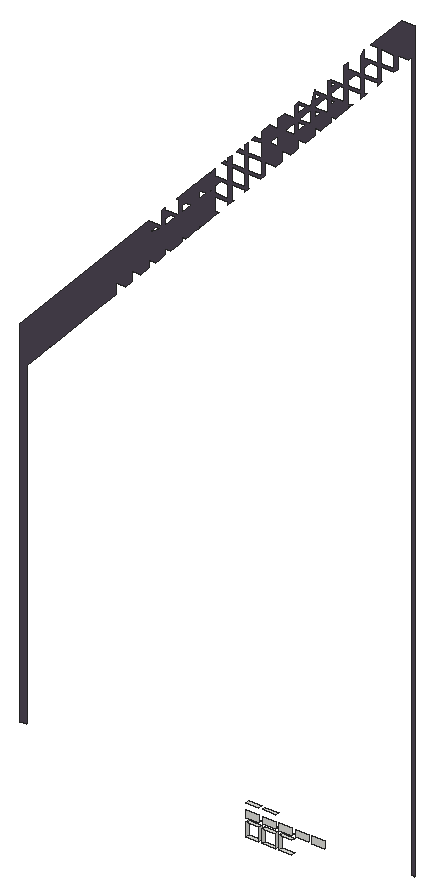
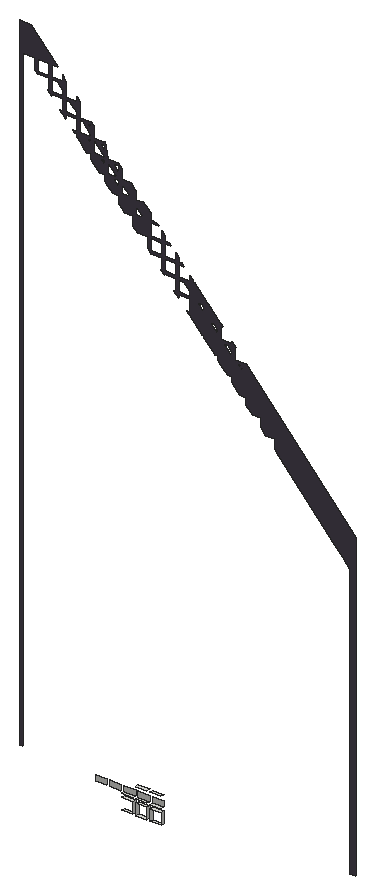
# SketchUp Ruby script. Lengths in inches.
U = 1.inch
M = Sketchup.active_model
def pt(a) = Geom::Point3d.new(a.map { |v| v * U })
def face(e, loops, mat)
  f = e.add_face(loops[0].map { |a| pt(a) })
  loops[1..].each { |l| e.add_face(l.map { |a| pt(a) }).erase! }
  f.material = f.back_material = mat if mat
  f
end
# faces: each face lists its corners as indices into pts; further lists are holes
def faces(e, pts, list, mat = nil) = list.each { |f| face(e, (f[0].is_a?(Array) ? f : [f]).map { |l| l.map { |i| pts[i] } }, mat) }
# xy, xz, yz: faces in a plane at the given z, y or x. An outline is a flat list of corners, or four numbers for a rectangle; further outlines are holes
def ring(l) = l.size == 4 ? [[l[0], l[1]], [l[2], l[1]], [l[2], l[3]], [l[0], l[3]]] : l.each_slice(2).to_a
def flat(e, list, mat, &to3) = list.each { |f| face(e, (f[0].is_a?(Array) ? f : [f]).map { |l| ring(l).map { |u, v| to3.(u, v) } }, mat) }
def xy(e, z, list, mat = nil) = flat(e, list, mat) { |x, y| [x, y, z] }
def xz(e, y, list, mat = nil) = flat(e, list, mat) { |x, z| [x, y, z] }
def yz(e, x, list, mat = nil) = flat(e, list, mat) { |y, z| [x, y, z] }
def lines(e, pts, list) = list.each { |a, b| e.add_line(pt(pts[a]), pt(pts[b])) }
# prism: a flat outline (further loops are holes) pulled along v
def prism(e, loops, v, mat = nil)
  f = face(e, loops, mat); d = Geom::Vector3d.new(v.map { |x| x * U })
  f.pushpull(f.normal.samedirection?(d) ? d.length : -d.length)
end
def box(e, o, s, mat = nil) = prism(e, [[o, [o[0] + s[0], o[1], o[2]], [o[0] + s[0], o[1] + s[1], o[2]], [o[0], o[1] + s[1], o[2]]]], [0, 0, s[2]], mat)
def at(x, y, z, deg = 0) = Geom::Transformation.translation(pt([x, y, z])) * Geom::Transformation.rotation(ORIGIN, Z_AXIS, deg.degrees)
def axes(o, x, y, z) = Geom::Transformation.new([*x, 0, *y, 0, *z, 0, *pt(o).to_a, 1])
def part(name) = M.definitions.add(name)
# library, detail: a bought-in or finely detailed component or shape, given as its bounding box
def library(name, o, s) = part(name).tap { |d| box(d.entities, o, s) }
def detail(e, o, s) = box(e.add_group.entities, o, s)
def put(e, d, t, mat = nil) = e.add_instance(d, t).tap { |i| i.material = mat if mat }
def group(e, t, mat = nil) = e.add_group.tap { |g| g.transformation = t; g.material = mat if mat }.entities
root = M.entities
M.materials.add("[Color M06]").color = [79, 71, 84]
xy(root,259.684,[[1357.054,480.141,1359.367,480.766],[1359.966,480.141,1362.279,480.766],[1362.879,480.141,1365.191,480.766]])
xy(root,261.996,[[1357.054,480.141,1359.367,480.766],[1359.966,480.141,1362.279,480.766],[1362.879,480.141,1365.191,480.766]])
xy(root,262.728,[[1357.083,480.141,1359.396,480.766],[1359.995,480.141,1362.308,480.766],[1362.908,480.141,1365.22,480.766]])
xy(root,265.041,[[1357.083,480.141,1359.396,480.766],[1359.995,480.141,1362.308,480.766]])
xz(root,480.141,[[1357.083,262.728,1359.396,263.889],[1359.995,262.728,1362.308,263.889],[1362.908,262.728,1365.22,263.889],[1365.82,262.728,1368.132,263.889],[1368.732,262.728,1371.044,263.889]])
xz(root,480.141,[[[1317.439,263.889,1318.577,263.889,1318.577,320.238,1319.662,321.395,1320.193,321.962,1322.574,324.502,1322.574,324.774,1322.829,324.774,1331.31,333.822,1333.374,336.024,1334.222,336.929,1334.222,338.837,1336.01,338.837,1337.134,340.036,1337.134,341.649,1338.646,341.649,1340.046,343.143,1340.046,344.462,1341.282,344.462,1341.751,344.962,1342.359,345.61,1342.958,346.25,1342.958,347.274,1343.918,347.274,1344.387,347.774,1345.271,348.717,1345.87,349.357,1345.87,350.087,1346.554,350.087,1347.023,350.587,1348.183,351.824,1348.782,352.464,1348.782,352.899,1349.19,352.899,1349.659,353.399,1351.095,354.931,1351.694,355.571,1351.694,355.712,1351.826,355.712,1352.295,356.212,1351.694,356.212,1351.694,358.524,1354.007,358.524,1354.007,358.038,1354.931,359.024,1354.606,359.024,1354.606,361.337,1356.919,361.337,1356.919,361.145,1357.567,361.837,1357.518,361.837,1357.518,364.149,1359.735,364.149,1360.43,364.891,1360.43,366.962,1362.371,366.962,1363.342,367.998,1363.342,369.774,1365.007,369.774,1365.476,370.274,1365.655,370.466,1366.254,371.105,1366.254,372.587,1367.643,372.587,1368.112,373.087,1368.567,373.573,1369.167,374.212,1369.167,375.399,1370.279,375.399,1370.689,375.837,1371.479,376.679,1372.079,377.319,1372.079,378.149,1372.857,378.149,1373.267,378.587,1374.391,379.786,1374.991,380.426,1374.991,380.899,1375.434,380.899,1375.844,381.337,1374.991,381.337,1374.991,383.649,1377.303,383.649,1377.303,382.893,1377.903,383.533,1377.903,383.649,1378.012,383.649,1378.101,383.746,1378.422,384.087,1377.903,384.087,1377.903,386.399,1380.215,386.399,1380.215,386,1380.999,386.837,1380.815,386.837,1380.815,389.149,1383.127,389.149,1383.127,389.107,1383.727,389.747,1383.727,391.899,1385.744,391.899,1386.175,392.359,1386.175,263.889,1386.751,263.889,1386.751,397.749,1384.501,397.749,1378.995,391.899,1380.215,391.899,1380.215,389.587,1377.903,389.587,1377.903,390.739,1377.303,390.102,1377.303,389.587,1376.818,389.587,1376.406,389.149,1377.303,389.149,1377.303,386.837,1374.991,386.837,1374.991,387.645,1374.391,387.008,1374.391,386.837,1374.229,386.837,1373.818,386.399,1374.391,386.399,1374.391,384.087,1372.079,384.087,1372.079,384.552,1371.229,383.649,1371.479,383.649,1371.479,381.337,1369.167,381.337,1369.167,381.458,1368.567,380.821,1368.567,378.587,1366.464,378.587,1365.655,377.727,1365.655,375.837,1363.875,375.837,1363.463,375.399,1363.342,375.271,1362.743,374.634,1362.743,373.087,1361.287,373.087,1360.816,372.587,1360.43,372.177,1359.831,371.54,1359.831,370.274,1358.639,370.274,1358.169,369.774,1359.831,369.774,1359.831,367.462,1357.518,367.462,1357.518,369.083,1356.919,368.447,1356.919,367.462,1355.992,367.462,1355.521,366.962,1356.919,366.962,1356.919,364.649,1354.606,364.649,1354.606,365.99,1354.007,365.353,1354.007,364.649,1353.344,364.649,1352.874,364.149,1354.007,364.149,1354.007,361.837,1351.694,361.837,1351.694,362.896,1351.095,362.259,1351.095,361.837,1350.697,361.837,1350.226,361.337,1348.782,359.803,1348.183,359.166,1348.183,359.024,1348.05,359.024,1347.579,358.524,1345.87,356.709,1344.932,355.712,1345.271,355.712,1345.271,353.399,1342.958,353.399,1342.958,353.615,1342.284,352.899,1342.359,352.899,1342.359,350.587,1340.107,350.587,1317.439,326.504],[1354.606,361.837,1356.919,364.149],[1357.518,364.649,1359.831,366.962],[1380.815,389.587,1383.127,391.899],[1377.903,386.837,1377.903,387.983,1379,389.149,1380.215,389.149,1380.215,386.837],[1351.694,359.024,1351.694,360.14,1352.82,361.337,1354.007,361.337,1354.007,359.024],[1374.991,384.087,1374.991,384.89,1376.412,386.399,1377.303,386.399,1377.303,384.087],[1372.079,381.337,1372.079,381.796,1373.823,383.649,1374.391,383.649,1374.391,381.337],[1369.167,378.587,1369.167,378.702,1371.234,380.899,1371.479,380.899,1371.479,378.587],[1366.469,375.837,1368.567,378.065,1368.567,375.837],[1340.046,347.774,1340.046,348.768,1341.282,350.087,1342.231,350.087,1340.054,347.774],[1363.881,373.087,1365.655,374.972,1365.655,373.087],[1342.958,350.86,1342.958,351.875,1343.918,352.899,1344.878,352.899],[1361.233,370.274,1362.743,371.878,1362.743,370.274],[1345.87,353.953,1345.87,354.982,1346.554,355.712,1347.526,355.712],[1366.254,373.918,1366.254,375.399,1367.643,375.399],[1366.254,376.668,1366.254,378.149,1367.643,378.149],[1348.782,357.047,1348.782,358.089,1349.19,358.524,1350.173,358.524],[1369.167,376.962,1369.167,378.149,1370.279,378.149],[1369.167,379.712,1369.167,380.899,1370.279,380.899],[1372.079,380.069,1372.079,380.899,1372.857,380.899],[1372.079,382.819,1372.079,383.649,1372.857,383.649],[1350.644,359.024,1351.095,359.504,1351.095,359.024],[1374.991,385.926,1374.991,386.399,1375.434,386.399],[1360.43,369.421,1360.43,369.774,1360.762,369.774],[1347.996,356.212,1348.183,356.41,1348.183,356.212],[1351.694,361.196,1351.694,361.337,1351.826,361.337],[1377.903,389.033,1377.903,389.149,1378.012,389.149],[1363.342,372.515,1363.342,372.587,1363.41,372.587]]],"[Color M06]")
yz(root,1357.054,[[480.141,259.684,480.766,261.996]])
yz(root,1359.367,[[480.141,259.684,480.766,261.996]])
yz(root,1359.966,[[480.141,259.684,480.766,261.996]])
yz(root,1362.279,[[480.141,259.684,480.766,261.996]])
yz(root,1362.879,[[480.141,259.684,480.766,261.996]])
